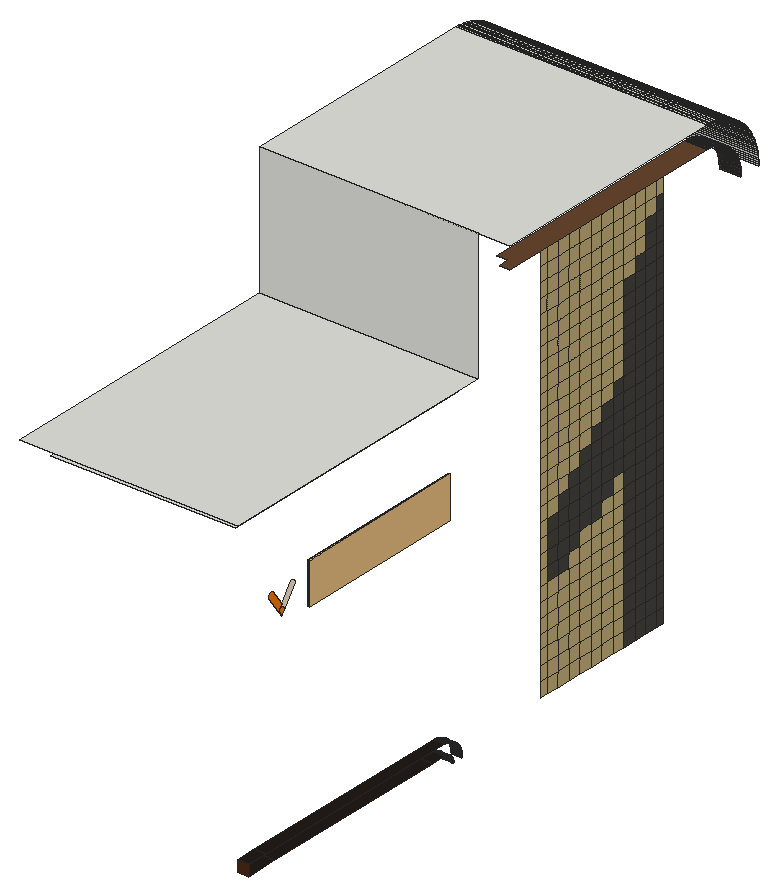
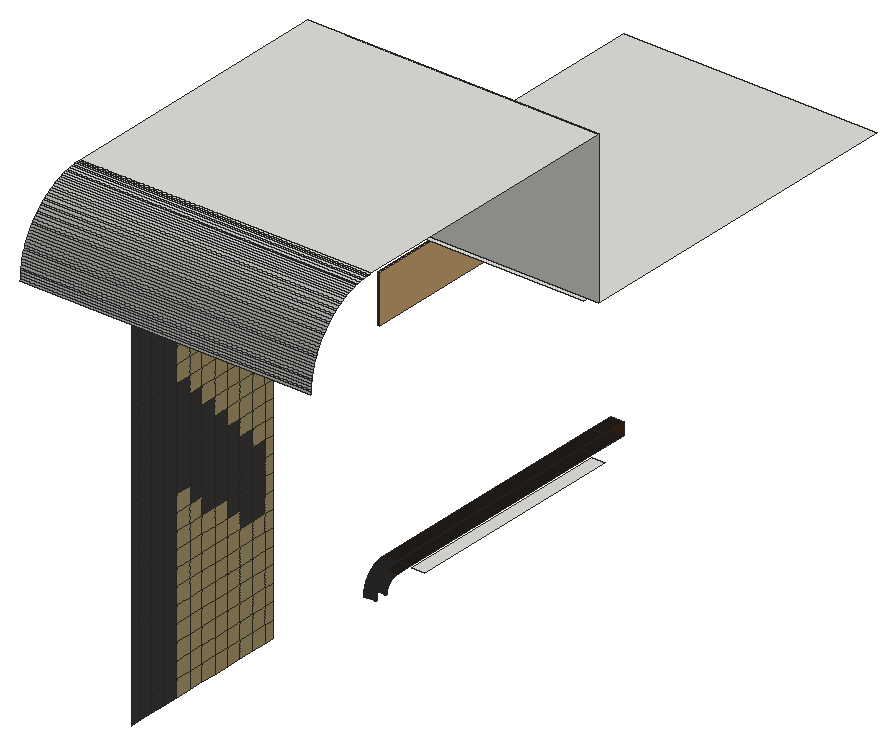
# SketchUp Ruby script. Lengths in inches.
U = 1.inch
M = Sketchup.active_model
def pt(a) = Geom::Point3d.new(a.map { |v| v * U })
def face(e, loops, mat)
  f = e.add_face(loops[0].map { |a| pt(a) })
  loops[1..].each { |l| e.add_face(l.map { |a| pt(a) }).erase! }
  f.material = f.back_material = mat if mat
  f
end
# faces: each face lists its corners as indices into pts; further lists are holes
def faces(e, pts, list, mat = nil) = list.each { |f| face(e, (f[0].is_a?(Array) ? f : [f]).map { |l| l.map { |i| pts[i] } }, mat) }
# xy, xz, yz: faces in a plane at the given z, y or x. An outline is a flat list of corners, or four numbers for a rectangle; further outlines are holes
def ring(l) = l.size == 4 ? [[l[0], l[1]], [l[2], l[1]], [l[2], l[3]], [l[0], l[3]]] : l.each_slice(2).to_a
def flat(e, list, mat, &to3) = list.each { |f| face(e, (f[0].is_a?(Array) ? f : [f]).map { |l| ring(l).map { |u, v| to3.(u, v) } }, mat) }
def xy(e, z, list, mat = nil) = flat(e, list, mat) { |x, y| [x, y, z] }
def xz(e, y, list, mat = nil) = flat(e, list, mat) { |x, z| [x, y, z] }
def yz(e, x, list, mat = nil) = flat(e, list, mat) { |y, z| [x, y, z] }
def lines(e, pts, list) = list.each { |a, b| e.add_line(pt(pts[a]), pt(pts[b])) }
# prism: a flat outline (further loops are holes) pulled along v
def prism(e, loops, v, mat = nil)
  f = face(e, loops, mat); d = Geom::Vector3d.new(v.map { |x| x * U })
  f.pushpull(f.normal.samedirection?(d) ? d.length : -d.length)
end
def box(e, o, s, mat = nil) = prism(e, [[o, [o[0] + s[0], o[1], o[2]], [o[0] + s[0], o[1] + s[1], o[2]], [o[0], o[1] + s[1], o[2]]]], [0, 0, s[2]], mat)
def at(x, y, z, deg = 0) = Geom::Transformation.translation(pt([x, y, z])) * Geom::Transformation.rotation(ORIGIN, Z_AXIS, deg.degrees)
def axes(o, x, y, z) = Geom::Transformation.new([*x, 0, *y, 0, *z, 0, *pt(o).to_a, 1])
def part(name) = M.definitions.add(name)
# library, detail: a bought-in or finely detailed component or shape, given as its bounding box
def library(name, o, s) = part(name).tap { |d| box(d.entities, o, s) }
def detail(e, o, s) = box(e.add_group.entities, o, s)
def put(e, d, t, mat = nil) = e.add_instance(d, t).tap { |i| i.material = mat if mat }
def group(e, t, mat = nil) = e.add_group.tap { |g| g.transformation = t; g.material = mat if mat }.entities
root = M.entities
M.materials.add("C01_Vanilla_Cream").color = [255, 230, 206]
M.materials.add("C05_Golden_Blaze").color = [255, 123, 0]
M.materials.add("Metal_10_1K").color = [196, 175, 123]
M.materials.add("Wood_Floor_12_1K").color = [35, 29, 25]
M.materials.add("Wood_Planks_01_1K").color = [69, 67, 63]
M.materials.add("Wood_Veneer_15_1K").color = [103, 69, 45]
M.materials.add("[Wood_Cherry_Original]1").color = [76, 43, 21]
c1 = library("CHOICE     HOLID",[0.51,0,0],[96.73,30.83,1])
xy(root,257,[[123,34,129,140.71]])
xy(root,257.99,[[129,150.24,135,150.34]],"Wood_Floor_12_1K")
xy(root,258,[[129,15,135,33],[129,33,135,141.71],[129,141.71,135,149.96],[129,149.96,135,150.05],[129,150.05,135,150.15]],"Wood_Floor_12_1K")
xy(root,263.99,[[129,150.34,135,150.52]],"Wood_Floor_12_1K")
xy(root,264,[[129,15,135,27],[129,27,135,149.96],[129,149.96,135,150.15]],"Wood_Floor_12_1K")
xy(root,423,[[21,21,123,174]])
xy(root,429,[[9,15,129,180]])
xy(root,489,[[141,180,141,186,135,186,135,315,147,315,147,180]],"Wood_Veneer_15_1K")
xy(root,501,[[9,180,147,315]])
xz(root,15,[[129,258,135,264]],"[Wood_Cherry_Original]1")
xz(root,155.95,[[129,252.28,135,252.375]],"Wood_Floor_12_1K")
xz(root,155.96,[[129,252,135,252.09],[129,252.09,135,252.1875]],"Wood_Floor_12_1K")
xz(root,161.95,[[129,252.375,135,252.57]],"Wood_Floor_12_1K")
xz(root,161.96,[[129,252,135,252.1875]],"Wood_Floor_12_1K")
xz(root,180,[[9,429,129,501]])
yz(root,129,[[45.07,371.33,45.26,371.58,43.14,374.47,43.02,374.3,42.96,374.22],[47.18,374.22,53.98,383.51,54.02,383.87,54,384.22,53.9,384.57,53.74,384.89,53.53,385.17,53.26,385.41,52.95,385.59,52.62,385.72,52.26,385.77,51.9,385.75,51.56,385.67,51.23,385.52,45.13,377.19,44.14,375.84,44.12,375.8,44.11,375.75,44.11,375.7,44.12,375.66,44.125,375.65,44.15,375.62,44.18,375.58,44.22,375.56,44.27,375.54,44.3125,375.54,44.36,375.56,44.4,375.58,44.44,375.61,45.35,376.73]],"C01_Vanilla_Cream")
yz(root,129,[[45.26,371.58,47.18,374.22,45.35,376.73,44.44,375.61,44.4,375.58,44.36,375.56,44.3125,375.54,44.27,375.54,44.22,375.56,44.18,375.58,44.15,375.62,44.125,375.65,44.12,375.66,44.11,375.7,44.11,375.75,44.12,375.8,44.14,375.84,43.14,374.47],[43.02,374.3,43.14,374.47,44.14,375.84,45.13,377.19,39.03,385.52,38.71,385.67,38.36,385.75,38,385.77,37.65,385.72,37.3125,385.59,37,385.41,36.74,385.17,36.52,384.89,36.36,384.57,36.27,384.22,36.24,383.87,36.28,383.51]],"C05_Golden_Blaze")
yz(root,135,[[216,257.625,220.5,265.5],[220.5,257.625,228,265.5],[228,257.625,235.5,265.5],[235.5,257.625,243,265.5],[243,257.625,250.5,265.5],
  [250.5,257.625,258,265.5],[258,257.625,265.5,265.5],[265.5,257.625,273,265.5],[216,265.5,220.5,273.375],[220.5,265.5,228,273.375],
  [228,265.5,235.5,273.375],[235.5,265.5,243,273.375],[243,265.5,250.5,273.375],[250.5,265.5,258,273.375],[258,265.5,265.5,273.375],
  [265.5,265.5,273,273.375],[216,273.375,220.5,281.25],[220.5,273.375,228,281.25],[228,273.375,235.5,281.25],[235.5,273.375,243,281.25],
  [243,273.375,250.5,281.25],[250.5,273.375,258,281.25],[258,273.375,265.5,281.25],[265.5,273.375,273,281.25],[216,281.25,220.5,289.125],
  [220.5,281.25,228,289.125],[228,281.25,235.5,289.125],[235.5,281.25,243,289.125],[243,281.25,250.5,289.125],[250.5,281.25,258,289.125],
  [258,281.25,265.5,289.125],[265.5,281.25,273,289.125],[216,289.125,220.5,297],[220.5,289.125,228,297],[228,289.125,235.5,297],
  [235.5,289.125,243,297],[243,289.125,250.5,297],[250.5,289.125,258,297],[258,289.125,265.5,297],[265.5,289.125,273,297],
  [216,297,220.5,304.875],[220.5,297,228,304.875],[228,297,235.5,304.875],[235.5,297,243,304.875],[243,297,250.5,304.875],
  [250.5,297,258,304.875],[258,297,265.5,304.875],[265.5,297,273,304.875],[216,304.875,220.5,312.75],[220.5,304.875,228,312.75],
  [228,304.875,235.5,312.75],[235.5,304.875,243,312.75],[243,304.875,250.5,312.75],[250.5,304.875,258,312.75],[258,304.875,265.5,312.75],
  [265.5,304.875,273,312.75],[216,312.75,220.5,320.625],[235.5,312.75,243,320.625],[243,312.75,250.5,320.625],[250.5,312.75,258,320.625],
  [258,312.75,265.5,320.625],[265.5,312.75,273,320.625],[216,320.625,220.5,328.5],[243,320.625,250.5,328.5],[250.5,320.625,258,328.5],
  [258,320.625,265.5,328.5],[265.5,320.625,273,328.5],[216,328.5,220.5,336.375],[258,328.5,265.5,336.375],[265.5,328.5,273,336.375],
  [216,336.375,220.5,344.25],[265.5,336.375,273,344.25],[216,344.25,220.5,352.125],[220.5,344.25,228,352.125],[216,352.125,220.5,360],
  [220.5,352.125,228,360],[228,352.125,235.5,360],[216,360,220.5,367.875],[220.5,360,228,367.875],[228,360,235.5,367.875],
  [235.5,360,243,367.875],[216,367.875,220.5,375.75],[220.5,367.875,228,375.75],[228,367.875,235.5,375.75],[235.5,367.875,243,375.75],
  [243,367.875,250.5,375.75],[216,375.75,220.5,383.625],[220.5,375.75,228,383.625],[228,375.75,235.5,383.625],[235.5,375.75,243,383.625],
  [243,375.75,250.5,383.625],[250.5,375.75,258,383.625],[216,383.625,220.5,391.5],[220.5,383.625,228,391.5],[228,383.625,235.5,391.5],
  [235.5,383.625,243,391.5],[243,383.625,250.5,391.5],[250.5,383.625,258,391.5],[258,383.625,265.5,391.5],[216,391.5,220.5,399.375],
  [220.5,391.5,228,399.375],[228,391.5,235.5,399.375],[235.5,391.5,243,399.375],[243,391.5,250.5,399.375],[250.5,391.5,258,399.375],
  [258,391.5,265.5,399.375],[265.5,391.5,273,399.375],[216,399.375,220.5,407.25],[220.5,399.375,228,407.25],[228,399.375,235.5,407.25],
  [235.5,399.375,243,407.25],[243,399.375,250.5,407.25],[250.5,399.375,258,407.25],[258,399.375,265.5,407.25],[265.5,399.375,273,407.25],
  [216,407.25,220.5,415.125],[220.5,407.25,228,415.125],[228,407.25,235.5,415.125],[235.5,407.25,243,415.125],[243,407.25,250.5,415.125],
  [250.5,407.25,258,415.125],[258,407.25,265.5,415.125],[265.5,407.25,273,415.125],[216,415.125,220.5,423],[220.5,415.125,228,423],
  [228,415.125,235.5,423],[235.5,415.125,243,423],[243,415.125,250.5,423],[250.5,415.125,258,423],[258,415.125,265.5,423],
  [265.5,415.125,273,423],[216,423,220.5,430.875],[220.5,423,228,430.875],[228,423,235.5,430.875],[235.5,423,243,430.875],
  [243,423,250.5,430.875],[250.5,423,258,430.875],[258,423,265.5,430.875],[265.5,423,273,430.875],[216,430.875,220.5,438.75],
  [220.5,430.875,228,438.75],[228,430.875,235.5,438.75],[235.5,430.875,243,438.75],[243,430.875,250.5,438.75],[250.5,430.875,258,438.75],
  [258,430.875,265.5,438.75],[265.5,430.875,273,438.75],[216,438.75,220.5,446.625],[220.5,438.75,228,446.625],[228,438.75,235.5,446.625],
  [235.5,438.75,243,446.625],[243,438.75,250.5,446.625],[250.5,438.75,258,446.625],[258,438.75,265.5,446.625],[265.5,438.75,273,446.625],
  [273,438.75,280.5,446.625],[216,446.625,220.5,454.5],[220.5,446.625,228,454.5],[228,446.625,235.5,454.5],[235.5,446.625,243,454.5],
  [243,446.625,250.5,454.5],[250.5,446.625,258,454.5],[258,446.625,265.5,454.5],[265.5,446.625,273,454.5],[273,446.625,280.5,454.5],
  [280.5,446.625,288,454.5],[216,454.5,220.5,462.375],[220.5,454.5,228,462.375],[228,454.5,235.5,462.375],[235.5,454.5,243,462.375],
  [243,454.5,250.5,462.375],[250.5,454.5,258,462.375],[258,454.5,265.5,462.375],[265.5,454.5,273,462.375],[273,454.5,280.5,462.375],
  [280.5,454.5,288,462.375],[216,462.375,220.5,470.25],[220.5,462.375,228,470.25],[228,462.375,235.5,470.25],[235.5,462.375,243,470.25],
  [243,462.375,250.5,470.25],[250.5,462.375,258,470.25],[258,462.375,265.5,470.25],[265.5,462.375,273,470.25],[273,462.375,280.5,470.25],
  [280.5,462.375,288,470.25],[288,462.375,295.5,470.25],[216,470.25,220.5,478.125],[220.5,470.25,228,478.125],[228,470.25,235.5,478.125],
  [235.5,470.25,243,478.125],[243,470.25,250.5,478.125],[250.5,470.25,258,478.125],[258,470.25,265.5,478.125],[265.5,470.25,273,478.125],
  [273,470.25,280.5,478.125],[280.5,470.25,288,478.125],[288,470.25,295.5,478.125],[295.5,470.25,300,478.125],[216,478.125,220.5,486],
  [220.5,478.125,228,486],[228,478.125,235.5,486],[235.5,478.125,243,486],[243,478.125,250.5,486],[250.5,478.125,258,486],
  [258,478.125,265.5,486],[265.5,478.125,273,486],[273,478.125,280.5,486],[280.5,478.125,288,486],[288,478.125,295.5,486],
  [295.5,478.125,300,486]],"Metal_10_1K")
yz(root,135,[[273,257.625,280.5,265.5],[280.5,257.625,288,265.5],[288,257.625,295.5,265.5],[295.5,257.625,300,265.5],[273,265.5,280.5,273.375],
  [280.5,265.5,288,273.375],[288,265.5,295.5,273.375],[295.5,265.5,300,273.375],[273,273.375,280.5,281.25],[280.5,273.375,288,281.25],
  [288,273.375,295.5,281.25],[295.5,273.375,300,281.25],[273,281.25,280.5,289.125],[280.5,281.25,288,289.125],[288,281.25,295.5,289.125],
  [295.5,281.25,300,289.125],[273,289.125,280.5,297],[280.5,289.125,288,297],[288,289.125,295.5,297],[295.5,289.125,300,297],
  [273,297,280.5,304.875],[280.5,297,288,304.875],[288,297,295.5,304.875],[295.5,297,300,304.875],[273,304.875,280.5,312.75],
  [280.5,304.875,288,312.75],[288,304.875,295.5,312.75],[295.5,304.875,300,312.75],[220.5,312.75,228,320.625],[228,312.75,235.5,320.625],
  [273,312.75,280.5,320.625],[280.5,312.75,288,320.625],[288,312.75,295.5,320.625],[295.5,312.75,300,320.625],[220.5,320.625,228,328.5],
  [228,320.625,235.5,328.5],[235.5,320.625,243,328.5],[273,320.625,280.5,328.5],[280.5,320.625,288,328.5],[288,320.625,295.5,328.5],
  [295.5,320.625,300,328.5],[220.5,328.5,228,336.375],[228,328.5,235.5,336.375],[235.5,328.5,243,336.375],[243,328.5,250.5,336.375],
  [250.5,328.5,258,336.375],[273,328.5,280.5,336.375],[280.5,328.5,288,336.375],[288,328.5,295.5,336.375],[295.5,328.5,300,336.375],
  [220.5,336.375,228,344.25],[228,336.375,235.5,344.25],[235.5,336.375,243,344.25],[243,336.375,250.5,344.25],[250.5,336.375,258,344.25],
  [258,336.375,265.5,344.25],[273,336.375,280.5,344.25],[280.5,336.375,288,344.25],[288,336.375,295.5,344.25],[295.5,336.375,300,344.25],
  [228,344.25,235.5,352.125],[235.5,344.25,243,352.125],[243,344.25,250.5,352.125],[250.5,344.25,258,352.125],[258,344.25,265.5,352.125],
  [265.5,344.25,273,352.125],[273,344.25,280.5,352.125],[280.5,344.25,288,352.125],[288,344.25,295.5,352.125],[295.5,344.25,300,352.125],
  [235.5,352.125,243,360],[243,352.125,250.5,360],[250.5,352.125,258,360],[258,352.125,265.5,360],[265.5,352.125,273,360],
  [273,352.125,280.5,360],[280.5,352.125,288,360],[288,352.125,295.5,360],[295.5,352.125,300,360],[243,360,250.5,367.875],
  [250.5,360,258,367.875],[258,360,265.5,367.875],[265.5,360,273,367.875],[273,360,280.5,367.875],[280.5,360,288,367.875],
  [288,360,295.5,367.875],[295.5,360,300,367.875],[250.5,367.875,258,375.75],[258,367.875,265.5,375.75],[265.5,367.875,273,375.75],
  [273,367.875,280.5,375.75],[280.5,367.875,288,375.75],[288,367.875,295.5,375.75],[295.5,367.875,300,375.75],[258,375.75,265.5,383.625],
  [265.5,375.75,273,383.625],[273,375.75,280.5,383.625],[280.5,375.75,288,383.625],[288,375.75,295.5,383.625],[295.5,375.75,300,383.625],
  [265.5,383.625,273,391.5],[273,383.625,280.5,391.5],[280.5,383.625,288,391.5],[288,383.625,295.5,391.5],[295.5,383.625,300,391.5],
  [273,391.5,280.5,399.375],[280.5,391.5,288,399.375],[288,391.5,295.5,399.375],[295.5,391.5,300,399.375],[273,399.375,280.5,407.25],
  [280.5,399.375,288,407.25],[288,399.375,295.5,407.25],[295.5,399.375,300,407.25],[273,407.25,280.5,415.125],[280.5,407.25,288,415.125],
  [288,407.25,295.5,415.125],[295.5,407.25,300,415.125],[273,415.125,280.5,423],[280.5,415.125,288,423],[288,415.125,295.5,423],
  [295.5,415.125,300,423],[273,423,280.5,430.875],[280.5,423,288,430.875],[288,423,295.5,430.875],[295.5,423,300,430.875],
  [273,430.875,280.5,438.75],[280.5,430.875,288,438.75],[288,430.875,295.5,438.75],[295.5,430.875,300,438.75],[280.5,438.75,288,446.625],
  [288,438.75,295.5,446.625],[295.5,438.75,300,446.625],[288,446.625,295.5,454.5],[295.5,446.625,300,454.5],[288,454.5,295.5,462.375],
  [295.5,454.5,300,462.375],[295.5,462.375,300,470.25]],"Wood_Planks_01_1K")
p = [[129,155.95,252.28],[129,155.96,252.1875],[135,155.96,252.1875],[135,155.95,252.28],[129,161.96,252.1875],[129,161.95,252.375],
  [135,161.95,252.375],[135,161.96,252.1875],[129,155.94,252.47],[129,155.95,252.375],[135,155.95,252.375],[135,155.94,252.47],
  [129,155.93,252.56],[135,155.93,252.56],[129,155.92,252.66],[135,155.92,252.66],[129,161.95,252.57],[129,161.9375,252.75],
  [135,161.9375,252.75],[135,161.95,252.57],[129,155.91,252.75],[135,155.91,252.75],[129,155.9,252.85],[135,155.9,252.85],
  [129,155.89,252.9375],[135,155.89,252.9375],[129,161.92,252.94],[135,161.92,252.94],[129,155.87,253.03],[135,155.87,253.03],
  [129,161.91,253.13],[135,161.91,253.13],[129,155.85,253.125],[135,155.85,253.125],[129,155.83,253.22],[135,155.83,253.22],
  [129,161.89,253.32],[135,161.89,253.32],[129,155.82,253.31],[135,155.82,253.31],[129,155.79,253.4],[135,155.79,253.4],
  [129,161.86,253.5],[135,161.86,253.5],[129,155.77,253.49],[135,155.77,253.49],[129,155.75,253.58],[135,155.75,253.58],
  [129,161.84,253.69],[135,161.84,253.69],[129,155.72,253.67],[135,155.72,253.67],[129,155.69,253.76],[135,155.69,253.76],
  [129,161.8125,253.88],[135,161.8125,253.88],[129,155.67,253.85],[135,155.67,253.85],[129,155.64,253.94],[135,155.64,253.94],
  [129,155.6,254.03],[135,155.6,254.03],[129,161.78,254.0625],[135,161.78,254.0625],[129,155.57,254.12],[135,155.57,254.12],
  [129,155.54,254.21],[135,155.54,254.21],[129,161.75,254.25],[135,161.75,254.25],[129,155.5,254.3],[135,155.5,254.3],
  [129,161.71,254.43],[135,161.71,254.43],[129,155.47,254.38],[135,155.47,254.38],[129,155.43,254.47],[135,155.43,254.47],
  [129,161.67,254.62],[135,161.67,254.62],[129,155.39,254.55],[135,155.39,254.55],[129,155.35,254.64],[135,155.35,254.64],
  [129,155.31,254.72],[135,155.31,254.72],[129,161.63,254.8],[135,161.63,254.8],[129,155.26,254.81],[135,155.26,254.81],
  [129,155.22,254.89],[135,155.22,254.89],[129,161.58,254.98],[135,161.58,254.98],[129,155.17,254.97],[135,155.17,254.97],
  [129,155.125,255.05],[135,155.125,255.05],[129,161.53,255.17],[135,161.53,255.17],[129,155.03,255.21],[129,155.08,255.13],
  [135,155.08,255.13],[135,155.03,255.21],[129,154.97,255.29],[135,154.97,255.29],[129,161.48,255.35],[135,161.48,255.35],
  [129,154.92,255.37],[135,154.92,255.37],[129,161.43,255.53],[135,161.43,255.53],[129,154.87,255.45],[135,154.87,255.45],
  [129,154.8125,255.53],[135,154.8125,255.53],[129,154.76,255.6],[135,154.76,255.6],[129,161.37,255.71],[135,161.37,255.71],
  [129,154.7,255.68],[135,154.7,255.68],[129,154.64,255.75],[135,154.64,255.75],[129,161.3125,255.89],[135,161.3125,255.89],
  [129,154.52,255.9],[129,154.58,255.82],[135,154.58,255.82],[135,154.52,255.9],[129,154.46,255.97],[135,154.46,255.97],
  [129,161.25,256.06],[135,161.25,256.06],[129,154.33,256.11],[129,154.4,256.04],[135,154.4,256.04],[135,154.33,256.11],
  [129,154.27,256.18],[135,154.27,256.18],[129,161.18,256.24],[135,161.18,256.24],[129,154.14,256.31],[129,154.2,256.24],
  [135,154.2,256.24],[135,154.14,256.31],[129,161.12,256.42],[135,161.12,256.42],[129,154.07,256.375],[135,154.07,256.375],
  [129,153.93,256.5],[129,154,256.4375],[135,154,256.4375],[135,153.93,256.5],[129,161.05,256.59],[135,161.05,256.59],
  [129,153.86,256.5625],[135,153.86,256.5625],[129,153.71,256.68],[129,153.78,256.625],[135,153.78,256.625],[135,153.71,256.68],
  [129,160.97,256.77],[135,160.97,256.77],[129,153.64,256.74],[135,153.64,256.74],[129,153.5625,256.8],[135,153.5625,256.8],
  [129,153.49,256.85],[135,153.49,256.85],[129,160.9,256.9375],[135,160.9,256.9375],[129,153.33,256.96],[129,153.41,256.91],
  [135,153.41,256.91],[135,153.33,256.96],[129,160.82,257.11],[135,160.82,257.11],[129,153.17,257.07],[129,153.25,257.01],
  [135,153.25,257.01],[135,153.17,257.07],[129,153.01,257.16],[129,153.09,257.12],[135,153.09,257.12],[135,153.01,257.16],
  [129,160.74,257.28],[135,160.74,257.28],[129,152.93,257.21],[135,152.93,257.21],[129,152.85,257.26],[135,152.85,257.26],
  [129,152.6,257.39],[129,152.68,257.35],[135,152.68,257.35],[135,152.6,257.39],[129,152.77,257.3],[135,152.77,257.3],
  [129,160.65,257.45],[135,160.65,257.45],[129,152.43,257.47],[129,152.51,257.43],[135,152.51,257.43],[135,152.43,257.47],
  [129,160.56,257.62],[135,160.56,257.62],[129,152.17,257.58],[129,152.26,257.54],[135,152.26,257.54],[135,152.17,257.58],
  [129,152.34,257.51],[135,152.34,257.51],[129,151.9,257.68],[129,151.99,257.65],[135,151.99,257.65],[135,151.9,257.68],
  [129,152.08,257.61],[135,152.08,257.61],[129,160.48,257.78],[135,160.48,257.78],[129,151.63,257.76],[129,151.72,257.73],
  [135,151.72,257.73],[135,151.63,257.76],[129,151.8125,257.71],[135,151.8125,257.71],[129,151.27,257.86],[129,151.36,257.83],
  [135,151.36,257.83],[135,151.27,257.86],[129,151.45,257.8125],[135,151.45,257.8125],[129,151.54,257.79],[135,151.54,257.79],
  [129,160.38,257.95],[135,160.38,257.95],[129,150.71,257.95],[129,150.8,257.94],[135,150.8,257.94],[135,150.71,257.95],
  [129,150.9,257.93],[135,150.9,257.93],[129,150.99,257.91],[135,150.99,257.91],[129,151.08,257.89],[135,151.08,257.89],
  [129,151.18,257.875],[135,151.18,257.875],[129,160.29,258.11],[135,160.29,258.11],[129,150.15,258],[129,150.24,257.99],
  [135,150.24,257.99],[135,150.15,258],[129,150.34,257.99],[129,150.43,257.98],[135,150.43,257.98],[135,150.34,257.99],
  [129,150.52,257.97],[135,150.52,257.97],[129,150.62,257.96],[135,150.62,257.96],[129,160.19,258.27],[135,160.19,258.27],
  [129,160.09,258.43],[135,160.09,258.43],[129,159.99,258.59],[135,159.99,258.59],[129,159.88,258.75],[135,159.88,258.75],
  [129,159.78,258.9],[135,159.78,258.9],[129,159.67,259.05],[135,159.67,259.05],[129,159.56,259.21],[135,159.56,259.21],
  [129,159.44,259.35],[135,159.44,259.35],[129,159.32,259.5],[135,159.32,259.5],[129,159.21,259.65],[135,159.21,259.65],
  [129,159.08,259.79],[135,159.08,259.79],[129,158.96,259.9375],[135,158.96,259.9375],[129,158.84,260.08],[135,158.84,260.08],
  [129,158.71,260.21],[135,158.71,260.21],[129,158.58,260.35],[135,158.58,260.35],[129,158.44,260.49],[135,158.44,260.49],
  [129,158.3125,260.62],[135,158.3125,260.62],[129,158.17,260.75],[135,158.17,260.75],[129,158.04,260.875],[135,158.04,260.875],
  [129,157.9,261],[135,157.9,261],[129,157.75,261.125],[135,157.75,261.125],[129,157.61,261.25],[135,157.61,261.25],
  [129,157.46,261.37],[135,157.46,261.37],[129,157.3125,261.48],[135,157.3125,261.48],[129,157.16,261.6],[135,157.16,261.6],
  [129,157.01,261.71],[135,157.01,261.71],[129,156.86,261.82],[135,156.86,261.82],[129,156.7,261.92],[135,156.7,261.92],
  [129,156.55,262.03],[135,156.55,262.03],[129,156.39,262.13],[135,156.39,262.13],[129,156.23,262.23],[135,156.23,262.23],
  [129,156.07,262.33],[135,156.07,262.33],[129,155.91,262.42],[135,155.91,262.42],[129,155.74,262.52],[135,155.74,262.52],
  [129,155.57,262.61],[135,155.57,262.61],[129,155.41,262.69],[135,155.41,262.69],[129,155.24,262.78],[135,155.24,262.78],
  [129,155.07,262.86],[135,155.07,262.86],[129,154.9,262.9375],[129,154.73,263.01],[135,154.73,263.01],[135,154.9,262.9375],
  [129,154.55,263.09],[135,154.55,263.09],[129,154.38,263.16],[135,154.38,263.16],[129,154.2,263.23],[129,154.02,263.29],
  [135,154.02,263.29],[135,154.2,263.23],[129,153.85,263.35],[135,153.85,263.35],[129,153.67,263.41],[129,153.49,263.47],
  [135,153.49,263.47],[135,153.67,263.41],[129,153.31,263.52],[129,153.125,263.57],[135,153.125,263.57],[135,153.31,263.52],
  [129,152.94,263.62],[129,152.76,263.67],[135,152.76,263.67],[135,152.94,263.62],[129,152.58,263.71],[129,152.39,263.75],
  [135,152.39,263.75],[135,152.58,263.71],[129,152.02,263.82],[129,151.84,263.85],[135,151.84,263.85],[135,152.02,263.82],
  [129,152.21,263.79],[135,152.21,263.79],[129,151.09,263.95],[129,150.9,263.96],[135,150.9,263.96],[135,151.09,263.95],
  [129,151.28,263.93],[135,151.28,263.93],[129,151.46,263.91],[135,151.46,263.91],[129,151.65,263.88],[135,151.65,263.88],
  [129,150.34,263.99],[129,150.15,264],[135,150.15,264],[135,150.34,263.99],[129,150.71,263.98],[129,150.52,263.99],
  [135,150.52,263.99],[135,150.71,263.98],[135,338.99,465.75],[135,339,465],[147,339,465],[147,338.99,465.75],
  [9,350.98,466.13],[147,350.98,466.13],[147,351,465],[9,351,465],[135,338.95,466.51],[147,338.95,466.51],
  [9,350.93,467.26],[147,350.93,467.26],[135,338.89,467.26],[147,338.89,467.26],[135,338.8125,468.01],[147,338.8125,468.01],
  [9,350.84,468.39],[147,350.84,468.39],[135,338.7,468.75],[147,338.7,468.75],[9,350.72,469.51],[147,350.72,469.51],
  [135,338.57,469.5],[147,338.57,469.5],[135,338.42,470.24],[147,338.42,470.24],[9,350.56,470.63],[147,350.56,470.63],
  [135,338.25,470.97],[147,338.25,470.97],[9,350.36,471.75],[147,350.36,471.75],[135,338.05,471.7],[147,338.05,471.7],
  [135,337.83,472.42],[147,337.83,472.42],[9,350.13,472.85],[147,350.13,472.85],[135,337.58,473.13],[147,337.58,473.13],
  [9,349.87,473.95],[147,349.87,473.95],[135,337.31,473.83],[147,337.31,473.83],[135,337.03,474.53],[147,337.03,474.53],
  [9,349.57,475.04],[147,349.57,475.04],[135,336.72,475.22],[147,336.72,475.22],[9,349.24,476.125],[147,349.24,476.125],
  [135,336.38,475.9],[147,336.38,475.9],[135,336.03,476.5625],[147,336.03,476.5625],[9,348.87,477.19],[147,348.87,477.19],
  [135,335.66,477.22],[147,335.66,477.22],[135,335.26,477.86],[147,335.26,477.86],[9,348.47,478.25],[147,348.47,478.25],
  [135,334.85,478.49],[147,334.85,478.49],[9,348.04,479.3],[147,348.04,479.3],[135,334.42,479.11],[147,334.42,479.11],
  [135,333.96,479.71],[147,333.96,479.71],[9,347.57,480.33],[147,347.57,480.33],[135,333.49,480.3],[147,333.49,480.3],
  [135,333,480.87],[147,333,480.87],[9,347.08,481.34],[147,347.08,481.34],[135,332.5,481.43],[147,332.5,481.43],
  [9,346.55,482.34],[147,346.55,482.34],[135,331.97,481.97],[147,331.97,481.97],[135,331.43,482.5],[147,331.43,482.5],
  [9,345.99,483.33],[147,345.99,483.33],[135,330.87,483],[147,330.87,483],[135,330.3,483.49],[147,330.3,483.49],
  [9,345.4,484.29],[147,345.4,484.29],[135,329.71,483.96],[147,329.71,483.96],[135,329.11,484.42],[147,329.11,484.42],
  [9,344.77,485.24],[147,344.77,485.24],[135,328.49,484.85],[147,328.49,484.85],[135,327.86,485.26],[147,327.86,485.26],
  [9,344.125,486.16],[147,344.125,486.16],[135,327.22,485.66],[147,327.22,485.66],[135,326.5625,486.03],[147,326.5625,486.03],
  [135,325.9,486.38],[147,325.9,486.38],[9,343.45,487.06],[147,343.45,487.06],[135,325.22,486.72],[147,325.22,486.72],
  [135,324.53,487.03],[147,324.53,487.03],[135,323.83,487.31],[147,323.83,487.31],[9,342.74,487.95],[147,342.74,487.95],
  [135,323.13,487.58],[147,323.13,487.58],[135,322.42,487.83],[147,322.42,487.83],[135,321.7,488.05],[147,321.7,488.05],
  [9,342,488.81],[147,342,488.81],[135,320.97,488.25],[147,320.97,488.25],[135,320.24,488.42],[147,320.24,488.42],
  [135,319.5,488.57],[147,319.5,488.57],[135,318.75,488.7],[147,318.75,488.7],[135,318.01,488.8125],[147,318.01,488.8125],
  [135,317.26,488.89],[147,317.26,488.89],[9,341.24,489.64],[147,341.24,489.64],[135,316.51,488.95],[147,316.51,488.95],
  [135,315,489],[135,315.75,488.99],[147,315.75,488.99],[147,315,489],[9,340.46,490.46],[147,340.46,490.46],
  [9,339.64,491.24],[147,339.64,491.24],[9,338.81,492],[147,338.81,492],[9,337.95,492.74],[147,337.95,492.74],
  [9,337.06,493.45],[147,337.06,493.45],[9,336.16,494.125],[147,336.16,494.125],[9,335.24,494.77],[147,335.24,494.77],
  [9,334.29,495.4],[147,334.29,495.4],[9,333.33,495.99],[147,333.33,495.99],[9,332.34,496.55],[147,332.34,496.55],
  [9,331.34,497.08],[147,331.34,497.08],[9,330.33,497.57],[147,330.33,497.57],[9,329.3,498.04],[147,329.3,498.04],
  [9,328.25,498.47],[147,328.25,498.47],[9,327.19,498.87],[147,327.19,498.87],[9,326.125,499.24],[147,326.125,499.24],
  [9,325.04,499.57],[147,325.04,499.57],[9,323.95,499.87],[147,323.95,499.87],[9,322.85,500.13],[147,322.85,500.13],
  [9,321.75,500.36],[147,321.75,500.36],[9,320.63,500.56],[147,320.63,500.56],[9,319.51,500.72],[147,319.51,500.72],
  [9,318.39,500.84],[147,318.39,500.84],[9,317.26,500.93],[147,317.26,500.93],[9,316.13,500.98],[147,316.13,500.98],
  [9,315,501],[147,315,501]]
faces(root,p,[[0,1,2,3],[4,5,6,7],[8,9,10,11],[12,8,11,13],[14,12,13,15],[16,17,18,19],[20,14,15,21],[22,20,21,23],
  [24,22,23,25],[17,26,27,18],[28,24,25,29],[26,30,31,27],[32,28,29,33],[34,32,33,35],[30,36,37,31],[38,34,35,39],
  [40,38,39,41],[36,42,43,37],[44,40,41,45],[46,44,45,47],[42,48,49,43],[50,46,47,51],[52,50,51,53],[48,54,55,49],
  [56,52,53,57],[58,56,57,59],[60,58,59,61],[54,62,63,55],[64,60,61,65],[66,64,65,67],[62,68,69,63],[70,66,67,71],
  [68,72,73,69],[74,70,71,75],[76,74,75,77],[72,78,79,73],[80,76,77,81],[82,80,81,83],[84,82,83,85],[78,86,87,79],
  [88,84,85,89],[90,88,89,91],[86,92,93,87],[94,90,91,95],[96,94,95,97],[92,98,99,93],[100,101,102,103],[101,96,97,102],
  [104,100,103,105],[98,106,107,99],[108,104,105,109],[106,110,111,107],[112,108,109,113],[114,112,113,115],[116,114,115,117],[110,118,119,111],
  [120,116,117,121],[122,120,121,123],[118,124,125,119],[126,127,128,129],[127,122,123,128],[130,126,129,131],[124,132,133,125],[134,135,136,137],
  [135,130,131,136],[138,134,137,139],[132,140,141,133],[142,143,144,145],[143,138,139,144],[140,146,147,141],[148,142,145,149],[150,151,152,153],
  [151,148,149,152],[146,154,155,147],[156,150,153,157],[158,159,160,161],[159,156,157,160],[154,162,163,155],[164,158,161,165],[166,164,165,167],
  [168,166,167,169],[162,170,171,163],[172,173,174,175],[173,168,169,174],[170,176,177,171],[178,179,180,181],[179,172,175,180],[182,183,184,185],
  [183,178,181,184],[176,186,187,177],[188,182,185,189],[190,188,189,191],[192,193,194,195],[193,196,197,194],[196,190,191,197],[186,198,199,187],
  [200,201,202,203],[201,192,195,202],[198,204,205,199],[206,207,208,209],[210,200,203,211],[207,210,211,208],[212,213,214,215],[213,216,217,214],
  [216,206,209,217],[204,218,219,205],[220,221,222,223],[221,224,225,222],[224,212,215,225],[226,227,228,229],[227,230,231,228],[232,220,223,233],
  [230,232,233,231],[218,234,235,219],[236,237,238,239],[237,240,241,238],[240,242,243,241],[242,244,245,243],[244,246,247,245],[246,226,229,247],
  [234,248,249,235],[250,251,252,253],[254,255,256,257],[255,258,259,256],[258,260,261,259],[260,236,239,261],[248,262,263,249],[262,264,265,263],
  [264,266,267,265],[266,268,269,267],[268,270,271,269],[270,272,273,271],[272,274,275,273],[274,276,277,275],[276,278,279,277],[278,280,281,279],
  [280,282,283,281],[282,284,285,283],[284,286,287,285],[286,288,289,287],[288,290,291,289],[290,292,293,291],[292,294,295,293],[294,296,297,295],
  [296,298,299,297],[298,300,301,299],[300,302,303,301],[302,304,305,303],[304,306,307,305],[306,308,309,307],[308,310,311,309],[310,312,313,311],
  [312,314,315,313],[314,316,317,315],[316,318,319,317],[318,320,321,319],[320,322,323,321],[322,324,325,323],[324,326,327,325],[326,328,329,327],
  [328,330,331,329],[330,332,333,331],[332,334,335,333],[334,336,337,335],[338,339,340,341],[336,338,341,337],[339,342,343,340],[342,344,345,343],
  [346,347,348,349],[344,346,349,345],[347,350,351,348],[352,353,354,355],[350,352,355,351],[356,357,358,359],[353,356,359,354],[360,361,362,363],
  [357,360,363,358],[364,365,366,367],[361,364,367,362],[368,369,370,371],[372,368,371,373],[365,372,373,366],[374,375,376,377],[378,374,377,379],
  [380,378,379,381],[382,380,381,383],[369,382,383,370],[384,385,386,387],[388,389,390,391],[375,388,391,376]],"Wood_Floor_12_1K")
faces(root,p,[[392,393,394,395],[400,392,395,401],[404,400,401,405],[406,404,405,407],[410,406,407,411],[414,410,411,415],[416,414,415,417],[420,416,417,421],
  [424,420,421,425],[426,424,425,427],[430,426,427,431],[434,430,431,435],[436,434,435,437],[440,436,437,441],[444,440,441,445],[446,444,445,447],
  [450,446,447,451],[452,450,451,453],[456,452,453,457],[460,456,457,461],[462,460,461,463],[466,462,463,467],[468,466,467,469],[472,468,469,473],
  [476,472,473,477],[478,476,477,479],[482,478,479,483],[484,482,483,485],[488,484,485,489],[490,488,489,491],[494,490,491,495],[496,494,495,497],
  [500,496,497,501],[502,500,501,503],[504,502,503,505],[508,504,505,509],[510,508,509,511],[512,510,511,513],[516,512,513,517],[518,516,517,519],
  [520,518,519,521],[524,520,521,525],[526,524,525,527],[528,526,527,529],[530,528,529,531],[532,530,531,533],[534,532,533,535],[538,534,535,539],
  [540,541,542,543],[541,538,539,542]],"Wood_Veneer_15_1K")
faces(root,p,[[396,397,398,399],[402,403,397,396],[408,409,403,402],[412,413,409,408],[418,419,413,412],[422,423,419,418],[428,429,423,422],[432,433,429,428],
  [438,439,433,432],[442,443,439,438],[448,449,443,442],[454,455,449,448],[458,459,455,454],[464,465,459,458],[470,471,465,464],[474,475,471,470],
  [480,481,475,474],[486,487,481,480],[492,493,487,486],[498,499,493,492],[506,507,499,498],[514,515,507,506],[522,523,515,514],[536,537,523,522],
  [544,545,537,536],[546,547,545,544],[548,549,547,546],[550,551,549,548],[552,553,551,550],[554,555,553,552],[556,557,555,554],[558,559,557,556],
  [560,561,559,558],[562,563,561,560],[564,565,563,562],[566,567,565,564],[568,569,567,566],[570,571,569,568],[572,573,571,570],[574,575,573,572],
  [576,577,575,574],[578,579,577,576],[580,581,579,578],[582,583,581,580],[584,585,583,582],[586,587,585,584],[588,589,587,586],[590,591,589,588],
  [592,593,591,590],[594,595,593,592]])
put(root,c1,axes([129,62.46,368.23],[0,1,0],[0,0,0.74],[1,0,0]),"C01_Vanilla_Cream")
